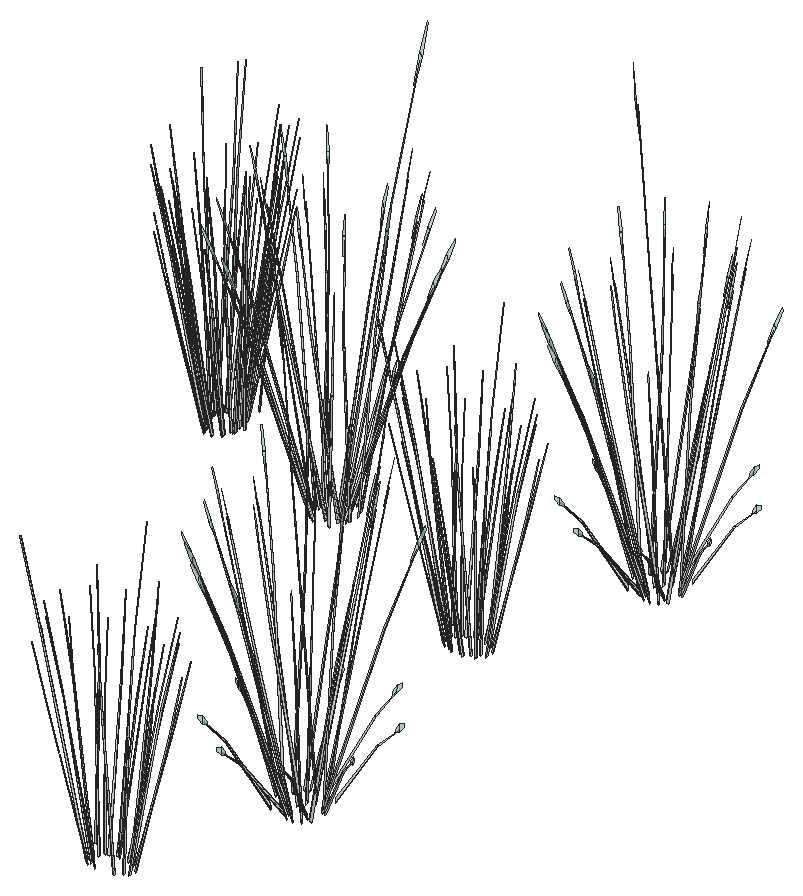
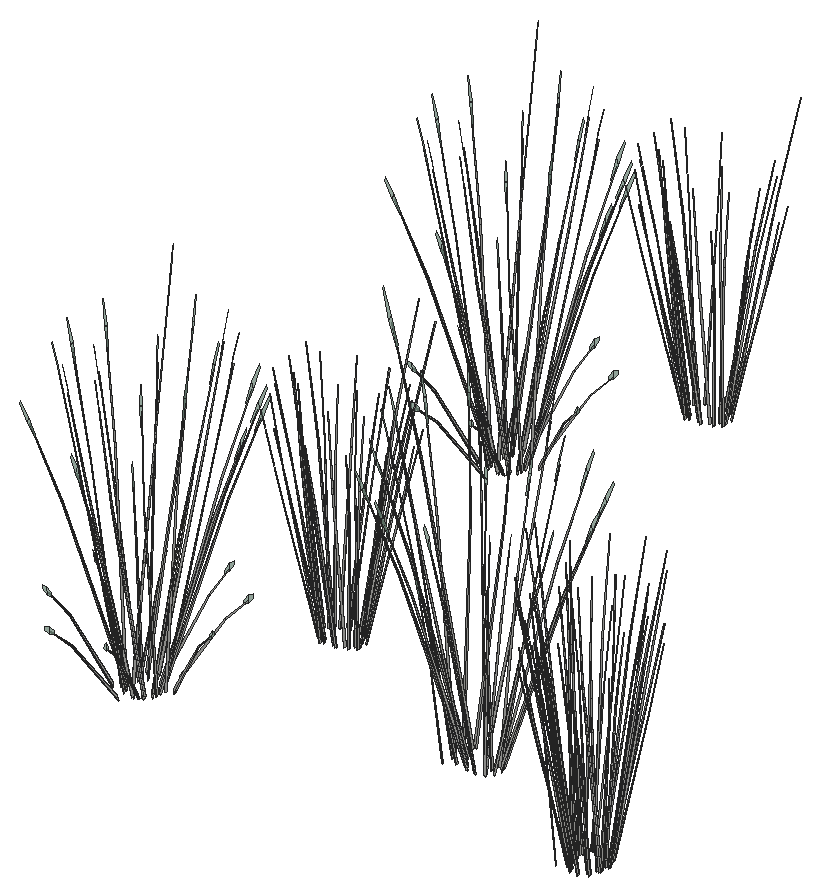
# SketchUp Ruby script. Lengths in inches.
U = 1.inch
M = Sketchup.active_model
def pt(a) = Geom::Point3d.new(a.map { |v| v * U })
def face(e, loops, mat)
  f = e.add_face(loops[0].map { |a| pt(a) })
  loops[1..].each { |l| e.add_face(l.map { |a| pt(a) }).erase! }
  f.material = f.back_material = mat if mat
  f
end
# faces: each face lists its corners as indices into pts; further lists are holes
def faces(e, pts, list, mat = nil) = list.each { |f| face(e, (f[0].is_a?(Array) ? f : [f]).map { |l| l.map { |i| pts[i] } }, mat) }
# xy, xz, yz: faces in a plane at the given z, y or x. An outline is a flat list of corners, or four numbers for a rectangle; further outlines are holes
def ring(l) = l.size == 4 ? [[l[0], l[1]], [l[2], l[1]], [l[2], l[3]], [l[0], l[3]]] : l.each_slice(2).to_a
def flat(e, list, mat, &to3) = list.each { |f| face(e, (f[0].is_a?(Array) ? f : [f]).map { |l| ring(l).map { |u, v| to3.(u, v) } }, mat) }
def xy(e, z, list, mat = nil) = flat(e, list, mat) { |x, y| [x, y, z] }
def xz(e, y, list, mat = nil) = flat(e, list, mat) { |x, z| [x, y, z] }
def yz(e, x, list, mat = nil) = flat(e, list, mat) { |y, z| [x, y, z] }
def lines(e, pts, list) = list.each { |a, b| e.add_line(pt(pts[a]), pt(pts[b])) }
# prism: a flat outline (further loops are holes) pulled along v
def prism(e, loops, v, mat = nil)
  f = face(e, loops, mat); d = Geom::Vector3d.new(v.map { |x| x * U })
  f.pushpull(f.normal.samedirection?(d) ? d.length : -d.length)
end
def box(e, o, s, mat = nil) = prism(e, [[o, [o[0] + s[0], o[1], o[2]], [o[0] + s[0], o[1] + s[1], o[2]], [o[0], o[1] + s[1], o[2]]]], [0, 0, s[2]], mat)
def at(x, y, z, deg = 0) = Geom::Transformation.translation(pt([x, y, z])) * Geom::Transformation.rotation(ORIGIN, Z_AXIS, deg.degrees)
def axes(o, x, y, z) = Geom::Transformation.new([*x, 0, *y, 0, *z, 0, *pt(o).to_a, 1])
def part(name) = M.definitions.add(name)
# library, detail: a bought-in or finely detailed component or shape, given as its bounding box
def library(name, o, s) = part(name).tap { |d| box(d.entities, o, s) }
def detail(e, o, s) = box(e.add_group.entities, o, s)
def put(e, d, t, mat = nil) = e.add_instance(d, t).tap { |i| i.material = mat if mat }
def group(e, t, mat = nil) = e.add_group.tap { |g| g.transformation = t; g.material = mat if mat }.entities
root = M.entities
M.materials.add("LightPink_Translucent").color = [175, 214, 192]
M.materials["LightPink_Translucent"].alpha = 0.75
c1 = part("blade")
p = [[2.15,0.21,22],[0,0.17,0],[0.09,0.45,0],[2.18,0.31,22],[2.29,0.31,22],[0.38,0.45,0],
  [2.48,0.24,33],[2.49,0.24,33],[2.48,0.22,33]]
faces(c1.entities,p,[[0,1,2,3],[4,5,2,3],[6,3,4,7],[8,0,3,6]])
c2 = part("blade with seeds\#1")
put(c2.entities,c1,at(0,0,0))
c3 = part("seeds")
p = [[0.3,-0.1,1.38],[-0.01,-0.03,1.59],[-0.01,-0.03,0.03],[0.14,-0.07,-0.07],[0.29,-0.03,3],[0.15,0.01,3.11]]
faces(c3.entities,p,[[0,1,2,3],[1,0,4,5]],"LightPink_Translucent")
c4 = part("blade with seeds")
put(c4.entities,c1,at(0,0,0))
put(c4.entities,c3,axes([2.4,0.25,30.99],[1.5799,-0.05474,1.17369],[-0.12525,1.92788,0.29478],[-0.07173,-0.02425,1.56792]))
put(root,c2,axes([487.46,499.57,140.86],[-0.33637,0.20062,0.29052],[-0.31842,-0.22908,-0.37506],[0.04845,-0.11639,0.71765]))
put(root,c2,axes([485.47,499.29,140.86],[0.07678,0.30692,0.29052],[-0.43892,0.08104,-0.37506],[-0.11789,-0.08795,0.71765]))
put(root,c2,axes([484.15,499.49,140.9],[0.41055,-0.28121,0.44104],[0.35407,0.29863,0.36366],[-0.19262,-0.05187,0.91263]))
put(root,c2,axes([484.34,499.49,140.6],[0.02503,-0.28975,0.05275],[0.378,0.00794,0.41527],[-0.1448,-0.03032,0.63322]))
put(root,c2,axes([488.05,500.19,140.86],[-0.43273,0.05446,0.29052],[-0.11427,-0.31131,-0.37506],[0.12401,-0.08362,0.71765]))
put(root,c2,axes([488.44,500.14,140.6],[0.34128,0.16025,0.05275],[-0.1987,0.22821,0.41527],[0.10942,-0.07378,0.63322]))
put(root,c2,axes([484.6,499.71,140.86],[0.28286,0.23857,0.29052],[-0.32298,0.22584,-0.37506],[-0.1641,-0.03436,0.71765]))
put(root,c2,axes([488.12,500.9375,140.86],[-0.41315,-0.1063,0.29052],[0.1205,-0.31012,-0.37506],[0.16634,-0.02844,0.71765]))
put(root,c2,axes([483.76,500.28,140.6],[-0.18259,-0.25981,0.05275],[0.33295,-0.12717,0.41527],[-0.14677,0.02509,0.63322]))
put(root,c2,axes([488.49,501.03,140.6],[0.18259,0.25981,0.05275],[-0.33295,0.12717,0.41527],[0.14677,-0.02509,0.63322]))
put(root,c2,axes([484.13,500.375,140.86],[0.41315,0.1063,0.29052],[-0.1205,0.31012,-0.37506],[-0.16634,0.02844,0.71765]))
put(root,c2,axes([487.65,501.61,140.86],[-0.28286,-0.23857,0.29052],[0.32298,-0.22584,-0.37506],[0.1641,0.03436,0.71765]))
put(root,c2,axes([483.81,501.17,140.6],[-0.34128,-0.16025,0.05275],[0.1987,-0.22821,0.41527],[-0.10942,0.07378,0.63322]))
put(root,c2,axes([484.2,501.12,140.86],[0.43273,-0.05446,0.29052],[0.11427,0.31131,-0.37506],[-0.12401,0.08362,0.71765]))
put(root,c2,axes([487.91,501.82,140.6],[-0.02503,0.28975,0.05275],[-0.378,-0.00794,0.41527],[0.1448,0.03032,0.63322]))
put(root,c2,axes([483.22,502,141.35],[0.43869,0.10171,-0.05322],[-0.13494,0.31305,-0.24131],[-0.07175,0.04753,0.79594]))
put(root,c2,axes([486.78,502.02,140.86],[-0.07678,-0.30692,0.29052],[0.43892,-0.08104,-0.37506],[0.11789,0.08795,0.71765]))
put(root,c2,axes([484.79,501.74,140.86],[0.33637,-0.20062,0.29052],[0.31842,0.22908,-0.37506],[-0.04845,0.11639,0.71765]))
put(root,c2,axes([484.48,501.92,140.6],[-0.40853,-0.01775,0.05275],[0.0112,-0.2681,0.41527],[-0.04275,0.1027,0.63322]))
put(root,c2,axes([485.73,502.07,140.86],[0.14987,-0.29303,0.29052],[0.43725,0.08547,-0.37506],[0.04009,0.11798,0.71765]))
put(root,c2,axes([486.85,502.3,140.6],[-0.22594,0.24206,0.05275],[-0.32175,-0.14093,0.41527],[0.10402,0.07761,0.63322]))
put(root,c2,axes([486.32,503.11,141.35],[0.34354,-0.2186,-0.05322],[0.31478,0.23941,-0.24131],[0.02216,0.06784,0.79594]))
put(root,c2,axes([485.59,502.33,140.6],[-0.36632,0.1295,0.05275],[-0.1793,-0.23615,0.41527],[0.03538,0.1041,0.63322]))
put(root,c2,axes([485.72,502.31,140.87],[-0.48986,-0.09962,0.43711],[0.16751,-0.3275,0.36041],[0.02944,0.12879,0.90448]))
put(root,c4,axes([493.6875,516.23,140.7],[0.01009,0.19824,1.55952],[-0.43714,-0.13151,0.1261],[0.02704,-0.28251,0.66668]))
put(root,c4,axes([492.92,516.3125,140.7],[0.0942,0.16583,1.55952],[-0.43527,0.13961,0.1261],[-0.09838,-0.26034,0.66668]))
put(root,c4,axes([493.07,515.81,141.46],[-0.05782,-0.07805,1.59199],[-0.42244,0.00664,-0.25177],[-0.05494,-0.1789,0.12768]))
put(root,c4,axes([494.39,516.61,140.7],[-0.07673,0.17753,1.55952],[-0.32188,-0.36739,0.1261],[0.14521,-0.22898,0.66668]))
put(root,c4,axes([495.1,516.57,141.46],[0.00314,-0.10283,1.59199],[-0.31434,-0.32739,-0.25177],[0.06423,-0.17468,0.12768]))
put(root,c4,axes([493.47,516.31,141.75],[-0.40325,0.24047,-0.11066],[-0.19816,-0.4268,-0.6142],[-0.0532,-0.17986,0.93327]))
put(root,c4,axes([494.3125,516.85,141.75],[-0.45289,-0.02559,-0.11066],[0.01238,-0.48454,-0.6142],[0.03146,-0.18661,0.93327]))
put(root,c4,axes([492.625,516.92,140.7],[0.13683,0.11937,1.55952],[-0.36934,0.30141,0.1261],[-0.1682,-0.20674,0.66668]))
put(root,c4,axes([492.29,516.83,140.7],[0.15307,0.08899,1.55952],[-0.31677,0.37333,0.1261],[-0.19743,-0.16841,0.66668]))
put(root,c4,axes([491.49,515.82,141.46],[-0.08813,-0.01188,1.59199],[-0.30658,0.33715,-0.25177],[-0.14498,-0.08826,0.12768]))
put(root,c4,axes([492.51,516.33,141.75],[-0.24556,0.44211,-0.11066],[-0.35561,-0.2547,-0.6142],[-0.12361,-0.12491,0.93327]))
put(root,c4,axes([494.83,517.34,140.7],[-0.14298,0.10925,1.55952],[-0.12037,-0.50484,0.1261],[0.22447,-0.1141,0.66668]))
put(root,c4,axes([495.78,518.17,141.46],[0.06244,-0.0731,1.59199],[-0.03959,-0.48785,-0.25177],[0.14934,-0.07786,0.12768]))
put(root,c4,axes([494.82,518.91,141.75],[-0.20734,-0.4677,-0.11066],[0.36799,-0.22984,-0.6142],[0.15507,-0.06171,0.93327]))
put(root,c4,axes([491.96,517.64,140.7],[0.17092,-0.0117,1.55952],[-0.11339,0.50701,0.1261],[-0.24358,-0.03136,0.66668]))
put(root,c4,axes([490.4,517.76,141.46],[-0.07171,0.06058,1.59199],[-0.02817,0.48891,-0.25177],[-0.15815,0.04916,0.12768]))
put(root,c4,axes([491.23,517.87,141.75],[0.20734,0.4677,-0.11066],[-0.36799,0.22984,-0.6142],[-0.15507,0.06171,0.93327]))
put(root,c4,axes([494.35,519.88,141.75],[0.02206,-0.52527,-0.11066],[0.41777,0.01436,-0.6142],[0.1609,0.03649,0.93327]))
put(root,c4,axes([492.04,518.54,140.7],[0.14298,-0.10925,1.55952],[0.12037,0.50484,0.1261],[-0.22447,0.1141,0.66668]))
put(root,c4,axes([493.49,519.3,141.24],[0.23139,-0.41299,1.25837],[0.36026,0.43608,0.54295],[-0.21711,0.13325,1.21634]))
put(root,c4,axes([495.02,520.36,141.46],[0.08863,-0.00461,1.59199],[0.25616,-0.38966,-0.25177],[0.15528,0.06024,0.12768]))
put(root,c4,axes([494.58,519.04,140.7],[-0.15307,-0.08899,1.55952],[0.31677,-0.37333,0.1261],[0.19743,0.16841,0.66668]))
put(root,c4,axes([491.24,518.98,141.75],[0.38119,0.2848,-0.11066],[-0.21961,0.41244,-0.6142],[-0.10769,0.14337,0.93327]))
put(root,c4,axes([493.53,520.46,141.75],[0.24556,-0.44211,-0.11066],[0.35561,0.2547,-0.6142],[0.12361,0.12491,0.93327]))
put(root,c4,axes([492.48,519.27,140.7],[0.07673,-0.17753,1.55952],[0.32188,0.36739,0.1261],[-0.14521,0.22898,0.66668]))
put(root,c4,axes([491.73,519.93,141.75],[0.45289,0.02559,-0.11066],[-0.01238,0.48454,-0.6142],[-0.03146,0.18661,0.93327]))
put(root,c4,axes([492.57,520.47,141.75],[0.40325,-0.24047,-0.11066],[0.19816,0.4268,-0.6142],[0.0532,0.17986,0.93327]))
put(root,c4,axes([492.01,520.36,141.46],[0.00753,0.10253,1.59199],[0.34598,0.28122,-0.25177],[-0.04567,0.18237,0.12768]))
put(root,c4,axes([493.18,519.64,140.7],[-0.01009,-0.19824,1.55952],[0.43714,0.13151,0.1261],[-0.02704,0.28251,0.66668]))
put(root,c4,axes([493.2,521.78,141.46],[0.06783,0.06632,1.59199],[0.4161,-0.08489,-0.25177],[0.07889,0.16641,0.12768]))
put(root,c2,axes([485.28,547.98,140.9],[0.55379,-0.09794,0.44104],[0.09611,0.38419,0.36366],[-0.13024,-0.11323,0.91263]))
put(root,c2,axes([486.66,548.03,140.6],[0.36632,-0.1295,0.05275],[0.1793,0.23615,0.41527],[-0.03538,-0.1041,0.63322]))
put(root,c2,axes([485.4,548.0625,140.6],[0.22594,-0.24206,0.05275],[0.32175,0.14093,0.41527],[-0.10402,-0.07761,0.63322]))
put(root,c2,axes([486.52,548.29,140.86],[-0.14987,0.29303,0.29052],[-0.43725,-0.08547,-0.37506],[-0.04009,-0.11798,0.71765]))
put(root,c2,axes([487.77,548.4375,140.6],[0.40853,0.01775,0.05275],[-0.0112,0.2681,0.41527],[0.04275,-0.1027,0.63322]))
put(root,c2,axes([487.46,548.62,140.86],[-0.33637,0.20062,0.29052],[-0.31842,-0.22908,-0.37506],[0.04845,-0.11639,0.71765]))
put(root,c2,axes([485.47,548.34,140.86],[0.07678,0.30692,0.29052],[-0.43892,0.08104,-0.37506],[-0.11789,-0.08795,0.71765]))
put(root,c2,axes([484.15,548.54,140.9],[0.41055,-0.28121,0.44104],[0.35407,0.29863,0.36366],[-0.19262,-0.05187,0.91263]))
put(root,c2,axes([484.34,548.54,140.6],[0.02503,-0.28975,0.05275],[0.378,0.00794,0.41527],[-0.1448,-0.03032,0.63322]))
put(root,c2,axes([488.05,549.24,140.86],[-0.43273,0.05446,0.29052],[-0.11427,-0.31131,-0.37506],[0.12401,-0.08362,0.71765]))
put(root,c2,axes([488.44,549.19,140.6],[0.34128,0.16025,0.05275],[-0.1987,0.22821,0.41527],[0.10942,-0.07378,0.63322]))
put(root,c2,axes([484.6,548.75,140.86],[0.28286,0.23857,0.29052],[-0.32298,0.22584,-0.37506],[-0.1641,-0.03436,0.71765]))
put(root,c2,axes([488.12,549.99,140.86],[-0.41315,-0.1063,0.29052],[0.1205,-0.31012,-0.37506],[0.16634,-0.02844,0.71765]))
put(root,c2,axes([483.76,549.33,140.6],[-0.18259,-0.25981,0.05275],[0.33295,-0.12717,0.41527],[-0.14677,0.02509,0.63322]))
put(root,c2,axes([488.49,550.08,140.6],[0.18259,0.25981,0.05275],[-0.33295,0.12717,0.41527],[0.14677,-0.02509,0.63322]))
put(root,c2,axes([484.13,549.42,140.86],[0.41315,0.1063,0.29052],[-0.1205,0.31012,-0.37506],[-0.16634,0.02844,0.71765]))
put(root,c2,axes([487.65,550.65,140.86],[-0.28286,-0.23857,0.29052],[0.32298,-0.22584,-0.37506],[0.1641,0.03436,0.71765]))
put(root,c2,axes([483.81,550.22,140.6],[-0.34128,-0.16025,0.05275],[0.1987,-0.22821,0.41527],[-0.10942,0.07378,0.63322]))
put(root,c2,axes([484.2,550.17,140.86],[0.43273,-0.05446,0.29052],[0.11427,0.31131,-0.37506],[-0.12401,0.08362,0.71765]))
put(root,c2,axes([487.91,550.87,140.6],[-0.02503,0.28975,0.05275],[-0.378,-0.00794,0.41527],[0.1448,0.03032,0.63322]))
put(root,c2,axes([483.22,551.05,141.35],[0.43869,0.10171,-0.05322],[-0.13494,0.31305,-0.24131],[-0.07175,0.04753,0.79594]))
put(root,c2,axes([486.78,551.07,140.86],[-0.07678,-0.30692,0.29052],[0.43892,-0.08104,-0.37506],[0.11789,0.08795,0.71765]))
put(root,c2,axes([484.79,550.79,140.86],[0.33637,-0.20062,0.29052],[0.31842,0.22908,-0.37506],[-0.04845,0.11639,0.71765]))
put(root,c2,axes([484.48,550.97,140.6],[-0.40853,-0.01775,0.05275],[0.0112,-0.2681,0.41527],[-0.04275,0.1027,0.63322]))
put(root,c2,axes([485.73,551.12,140.86],[0.14987,-0.29303,0.29052],[0.43725,0.08547,-0.37506],[0.04009,0.11798,0.71765]))
put(root,c2,axes([486.85,551.35,140.6],[-0.22594,0.24206,0.05275],[-0.32175,-0.14093,0.41527],[0.10402,0.07761,0.63322]))
put(root,c2,axes([486.32,552.16,141.35],[0.34354,-0.2186,-0.05322],[0.31478,0.23941,-0.24131],[0.02216,0.06784,0.79594]))
put(root,c2,axes([485.59,551.38,140.6],[-0.36632,0.1295,0.05275],[-0.1793,-0.23615,0.41527],[0.03538,0.1041,0.63322]))
put(root,c2,axes([485.72,551.36,140.87],[-0.48986,-0.09962,0.43711],[0.16751,-0.3275,0.36041],[0.02944,0.12879,0.90448]))
put(root,c4,axes([462.24,558.24,140.79],[0.10925,0.14298,1.55952],[-0.50484,0.12037,0.1261],[-0.1141,-0.22447,0.66668]))
put(root,c4,axes([463.95,558.49,140.79],[-0.08899,0.15307,1.55952],[-0.37333,-0.31677,0.1261],[0.16841,-0.19743,0.66668]))
put(root,c4,axes([463.82,558.25,141.85],[-0.4677,0.20734,-0.11066],[-0.22984,-0.36799,-0.6142],[-0.06171,-0.15507,0.93327]))
put(root,c4,axes([464.79,558.72,141.85],[-0.52527,-0.02206,-0.11066],[0.01436,-0.41777,-0.6142],[0.03649,-0.1609,0.93327]))
put(root,c4,axes([461.51,558.68,140.79],[0.17753,0.07673,1.55952],[-0.36739,0.32188,0.1261],[-0.22898,-0.14521,0.66668]))
put(root,c4,axes([465.36,559.54,141.85],[-0.44211,-0.24556,-0.11066],[0.2547,-0.35561,-0.6142],[0.12491,-0.12361,0.93327]))
put(root,c4,axes([461.75,558.76,141.85],[-0.02559,0.45289,-0.11066],[-0.48454,-0.01238,-0.6142],[-0.18661,-0.03146,0.93327]))
put(root,c4,axes([465.38,560.5,141.85],[-0.24047,-0.40325,-0.11066],[0.4268,-0.19816,-0.6142],[0.17986,-0.0532,0.93327]))
put(root,c4,axes([461.14,559.38,140.79],[0.19824,-0.01009,1.55952],[-0.13151,0.43714,0.1261],[-0.28251,-0.02704,0.66668]))
put(root,c4,axes([464.55,559.89,140.79],[-0.19824,0.01009,1.55952],[0.13151,-0.43714,0.1261],[0.28251,0.02704,0.66668]))
put(root,c4,axes([493.6875,565.28,140.7],[0.01009,0.19824,1.55952],[-0.43714,-0.13151,0.1261],[0.02704,-0.28251,0.66668]))
put(root,c4,axes([492.92,565.36,140.7],[0.0942,0.16583,1.55952],[-0.43527,0.13961,0.1261],[-0.09838,-0.26034,0.66668]))
put(root,c4,axes([461.21,559.6,141.85],[0.24047,0.40325,-0.11066],[-0.4268,0.19816,-0.6142],[-0.17986,0.0532,0.93327]))
put(root,c4,axes([465.96,561.35,140.84],[-0.09148,-0.37435,-0.03177],[0.43236,-0.08606,-0.14407],[0.09029,0.02373,0.47519]))
put(root,c4,axes([464.84,561.34,141.85],[0.02559,-0.45289,-0.11066],[0.48454,0.01238,-0.6142],[0.18661,0.03146,0.93327]))
put(root,c4,axes([493.07,564.86,141.46],[-0.05782,-0.07805,1.59199],[-0.42244,0.00664,-0.25177],[-0.05494,-0.1789,0.12768]))
put(root,c4,axes([494.39,565.65,140.7],[-0.07673,0.17753,1.55952],[-0.32188,-0.36739,0.1261],[0.14521,-0.22898,0.66668]))
put(root,c4,axes([461.22,560.15,140.79],[0.16583,-0.0942,1.55952],[0.13961,0.43527,0.1261],[-0.26034,0.09838,0.66668]))
put(root,c2,axes([445.85,564.61,140.7],[0.34743,0.14045,0.39379],[-0.1188,0.46175,0.3247],[-0.02088,-0.18159,0.81485]))
put(root,c2,axes([445.94,564.58,140.69],[0.25981,-0.18259,0.05275],[0.12717,0.33295,0.41527],[-0.02509,-0.14677,0.63322]))
put(root,c4,axes([495.1,565.62,141.46],[0.00314,-0.10283,1.59199],[-0.31434,-0.32739,-0.25177],[0.06423,-0.17468,0.12768]))
put(root,c4,axes([493.47,565.36,141.75],[-0.40325,0.24047,-0.11066],[-0.19816,-0.4268,-0.6142],[-0.0532,-0.17986,0.93327]))
put(root,c2,axes([444.98,564.72,140.7],[0.35069,-0.12329,0.39379],[0.06086,0.48364,0.3247],[-0.08248,-0.14254,0.81485]))
put(root,c4,axes([494.3125,565.9,141.75],[-0.45289,-0.02559,-0.11066],[0.01238,-0.48454,-0.6142],[0.03146,-0.18661,0.93327]))
put(root,c2,axes([445.05,564.63,140.69],[0.16025,-0.34128,0.05275],[0.22821,0.1987,0.41527],[-0.07378,-0.10942,0.63322]))
put(root,c4,axes([492.625,565.97,140.7],[0.13683,0.11937,1.55952],[-0.36934,0.30141,0.1261],[-0.1682,-0.20674,0.66668]))
put(root,c2,axes([445.84,564.95,140.96],[-0.1063,0.41315,0.29052],[-0.31012,-0.1205,-0.37506],[-0.02844,-0.16634,0.71765]))
put(root,c2,axes([446.64,565.13,140.7],[0.25108,0.36656,0.39379],[-0.26664,0.31614,0.3247],[0.04631,-0.17198,0.81485]))
put(root,c2,axes([446.73,565.16,140.69],[0.28975,0.02503,0.05275],[-0.00794,0.378,0.41527],[0.03032,-0.1448,0.63322]))
put(root,c2,axes([446.51,565.42,140.96],[-0.23857,0.28286,0.29052],[-0.22584,-0.32298,-0.37506],[0.03436,-0.1641,0.71765]))
put(root,c4,axes([492.29,565.88,140.7],[0.15307,0.08899,1.55952],[-0.31677,0.37333,0.1261],[-0.19743,-0.16841,0.66668]))
put(root,c4,axes([464.18,560.59,140.79],[-0.17753,-0.07673,1.55952],[0.36739,-0.32188,0.1261],[0.22898,0.14521,0.66668]))
put(root,c4,axes([464.21,559.58,141.34],[-0.41299,-0.23139,1.25837],[0.43608,-0.36026,0.54295],[0.13325,0.21711,1.21634]))
put(root,c4,axes([461.23,560.56,141.85],[0.44211,0.24556,-0.11066],[-0.2547,0.35561,-0.6142],[-0.12491,0.12361,0.93327]))
put(root,c4,axes([463.89,561.83,141.85],[0.2848,-0.38119,-0.11066],[0.41244,0.21961,-0.6142],[0.14337,0.10769,0.93327]))
put(root,c4,axes([491.49,564.87,141.46],[-0.08813,-0.01188,1.59199],[-0.30658,0.33715,-0.25177],[-0.14498,-0.08826,0.12768]))
put(root,c4,axes([461.83,560.45,140.79],[0.11937,-0.13683,1.55952],[0.30141,0.36934,0.1261],[-0.20674,0.1682,0.66668]))
put(root,c2,axes([445.1,565.02,140.96],[0.05446,0.43273,0.29052],[-0.31131,0.11427,-0.37506],[-0.08362,-0.12401,0.71765]))
put(root,c4,axes([492.51,565.375,141.75],[-0.24556,0.44211,-0.11066],[-0.35561,-0.2547,-0.6142],[-0.12361,-0.12491,0.93327]))
put(root,c2,axes([444.27,565.43,140.7],[0.25999,-0.354,0.39379],[0.22422,0.37594,0.3247],[-0.12198,-0.0653,0.81485]))
put(root,c2,axes([444.3,565.3,140.69],[0.01775,-0.40853,0.05275],[0.2681,0.0112,0.41527],[-0.1027,-0.04275,0.63322]))
put(root,c4,axes([461.74,560.78,140.79],[0.08899,-0.15307,1.55952],[0.37333,0.31677,0.1261],[-0.16841,0.19743,0.66668]))
put(root,c2,axes([446.93,566.29,140.96],[-0.30692,0.07678,0.29052],[-0.08104,-0.43892,-0.37506],[0.08795,-0.11789,0.71765]))
put(root,c4,axes([494.83,566.39,140.7],[-0.14298,0.10925,1.55952],[-0.12037,-0.50484,0.1261],[0.22447,-0.1141,0.66668]))
put(root,c4,axes([462.78,561.84,141.85],[0.4677,-0.20734,-0.11066],[0.22984,0.36799,-0.6142],[0.06171,0.15507,0.93327]))
put(root,c2,axes([447.14,566.13,140.7],[0.08745,0.49445,0.39379],[-0.34303,0.08581,0.3247],[0.1011,-0.11629,0.81485]))
put(root,c4,axes([463.44,561.04,140.79],[-0.10925,-0.14298,1.55952],[0.50484,-0.12037,0.1261],[0.1141,0.22447,0.66668]))
put(root,c2,axes([447.21,566.22,140.69],[0.24206,0.22594,0.05275],[-0.14093,0.32175,0.41527],[0.07761,-0.10402,0.63322]))
put(root,c4,axes([462.55,561.11,140.79],[-0.0117,-0.17092,1.55952],[0.50701,0.11339,0.1261],[-0.03136,0.24358,0.66668]))
put(root,c2,axes([444.48,565.61,140.96],[0.20062,0.33637,0.29052],[-0.22908,0.31842,-0.37506],[-0.11639,-0.04845,0.71765]))
put(root,c4,axes([495.78,567.22,141.46],[0.06244,-0.0731,1.59199],[-0.03959,-0.48785,-0.25177],[0.14934,-0.07786,0.12768]))
put(root,c2,axes([448.02,566.75,141.44],[-0.2186,-0.34354,-0.05322],[0.23941,-0.31478,-0.24131],[0.06784,-0.02216,0.79594]))
put(root,c4,axes([494.82,567.96,141.75],[-0.20734,-0.4677,-0.11066],[0.36799,-0.22984,-0.6142],[0.15507,-0.06171,0.93327]))
put(root,c4,axes([491.96,566.69,140.7],[0.17092,-0.0117,1.55952],[-0.11339,0.50701,0.1261],[-0.24358,-0.03136,0.66668]))
put(root,c2,axes([446.98,567.34,140.96],[-0.29303,-0.14987,0.29052],[0.08547,-0.43725,-0.37506],[0.11798,-0.04009,0.71765]))
put(root,c2,axes([443.91,566.54,140.7],[0.09962,-0.48986,0.39379],[0.3275,0.16751,0.3247],[-0.12879,0.02944,0.81485]))
put(root,c2,axes([443.88,566.41,140.69],[-0.1295,-0.36632,0.05275],[0.23615,-0.1793,0.41527],[-0.1041,0.03538,0.63322]))
put(root,c2,axes([447.24,567.48,140.69],[0.1295,0.36632,0.05275],[-0.23615,0.1793,0.41527],[0.1041,-0.03538,0.63322]))
put(root,c2,axes([447.22,567.35,140.97],[-0.09962,0.48986,0.43711],[-0.3275,-0.16751,0.36041],[0.12879,-0.02944,0.90448]))
put(root,c2,axes([444.15,566.55,140.96],[0.29303,0.14987,0.29052],[-0.08547,0.43725,-0.37506],[-0.11798,0.04009,0.71765]))
put(root,c4,axes([490.4,566.81,141.46],[-0.07171,0.06058,1.59199],[-0.02817,0.48891,-0.25177],[-0.15815,0.04916,0.12768]))
put(root,c2,axes([446.7,568.5,141.24],[0.01888,-0.54637,-0.11073],[0.35746,0.01493,-0.6146],[0.13767,0.03795,0.93387]))
put(root,c2,axes([446.65,568.29,140.96],[-0.20062,-0.33637,0.29052],[0.22908,-0.31842,-0.37506],[0.11639,0.04845,0.71765]))
put(root,c4,axes([491.23,566.92,141.75],[0.20734,0.4677,-0.11066],[-0.36799,0.22984,-0.6142],[-0.15507,0.06171,0.93327]))
put(root,c4,axes([494.35,568.93,141.75],[0.02206,-0.52527,-0.11066],[0.41777,0.01436,-0.6142],[0.1609,0.03649,0.93327]))
put(root,c2,axes([443.92,567.67,140.69],[-0.24206,-0.22594,0.05275],[0.14093,-0.32175,0.41527],[-0.07761,0.10402,0.63322]))
put(root,c2,axes([443.84,567.8,140.99],[-0.09794,-0.55379,0.44104],[0.38419,-0.09611,0.36366],[-0.11323,0.13024,0.91263]))
put(root,c2,axes([444.2,567.6,140.96],[0.30692,-0.07678,0.29052],[0.08104,0.43892,-0.37506],[-0.08795,0.11789,0.71765]))
put(root,c4,axes([492.04,567.59,140.7],[0.14298,-0.10925,1.55952],[0.12037,0.50484,0.1261],[-0.22447,0.1141,0.66668]))
put(root,c2,axes([446.83,568.59,140.69],[-0.01775,0.40853,0.05275],[-0.2681,-0.0112,0.41527],[0.1027,0.04275,0.63322]))
put(root,c2,axes([446.85,568.46,140.7],[-0.25999,0.354,0.39379],[-0.22422,-0.37594,0.3247],[0.12198,0.0653,0.81485]))
put(root,c4,axes([493.49,568.35,141.24],[0.23139,-0.41299,1.25837],[0.36026,0.43608,0.54295],[-0.21711,0.13325,1.21634]))
put(root,c2,axes([446.03,568.87,140.96],[-0.05446,-0.43273,0.29052],[0.31131,-0.11427,-0.37506],[0.08362,0.12401,0.71765]))
put(root,c4,axes([495.02,569.41,141.46],[0.08863,-0.00461,1.59199],[0.25616,-0.38966,-0.25177],[0.15528,0.06024,0.12768]))
put(root,c2,axes([446.91,569.85,141.44],[0.10171,-0.43869,-0.05322],[0.31305,0.13494,-0.24131],[0.04753,0.07175,0.79594]))
put(root,c2,axes([443.89,567.57,141.27],[0.3653,0.33178,-0.11173],[-0.21045,0.48049,-0.62013],[-0.10321,0.16702,0.94228]))
put(root,c2,axes([444.61,568.47,140.96],[0.23857,-0.28286,0.29052],[0.22584,0.32298,-0.37506],[-0.03436,0.1641,0.71765]))
put(root,c4,axes([494.58,568.09,140.7],[-0.15307,-0.08899,1.55952],[0.31677,-0.37333,0.1261],[0.19743,0.16841,0.66668]))
put(root,c2,axes([444.4,568.73,140.69],[-0.28975,-0.02503,0.05275],[0.00794,-0.378,0.41527],[-0.03032,0.1448,0.63322]))
put(root,c4,axes([491.24,568.03,141.75],[0.38119,0.2848,-0.11066],[-0.21961,0.41244,-0.6142],[-0.10769,0.14337,0.93327]))
put(root,c4,axes([493.53,569.51,141.75],[0.24556,-0.44211,-0.11066],[0.35561,0.2547,-0.6142],[0.12361,0.12491,0.93327]))
put(root,c2,axes([445.28,568.9375,140.96],[0.1063,-0.41315,0.29052],[0.31012,0.1205,-0.37506],[0.02844,0.16634,0.71765]))
put(root,c2,axes([446.07,569.26,140.69],[-0.16025,0.34128,0.05275],[-0.22821,-0.1987,0.41527],[0.07378,0.10942,0.63322]))
put(root,c2,axes([444.4,568.92,140.99],[-0.28121,-0.41055,0.44104],[0.29863,-0.35407,0.36366],[-0.05187,0.19262,0.91263]))
put(root,c2,axes([446.14,569.17,140.7],[-0.35069,0.12329,0.39379],[-0.06086,-0.48364,0.3247],[0.08248,0.14254,0.81485]))
put(root,c2,axes([445.18,569.3125,140.69],[-0.25981,0.18259,0.05275],[-0.12717,-0.33295,0.41527],[0.02509,0.14677,0.63322]))
put(root,c2,axes([445.28,569.28,140.7],[-0.34743,-0.14045,0.39379],[0.1188,-0.46175,0.3247],[0.02088,0.18159,0.81485]))
put(root,c4,axes([492.48,568.32,140.7],[0.07673,-0.17753,1.55952],[0.32188,0.36739,0.1261],[-0.14521,0.22898,0.66668]))
put(root,c4,axes([491.73,568.98,141.75],[0.45289,0.02559,-0.11066],[-0.01238,0.48454,-0.6142],[-0.03146,0.18661,0.93327]))
put(root,c4,axes([492.57,569.52,141.75],[0.40325,-0.24047,-0.11066],[0.19816,0.4268,-0.6142],[0.0532,0.17986,0.93327]))
put(root,c4,axes([492.01,569.4,141.46],[0.00753,0.10253,1.59199],[0.34598,0.28122,-0.25177],[-0.04567,0.18237,0.12768]))
put(root,c4,axes([493.18,568.69,140.7],[-0.01009,-0.19824,1.55952],[0.43714,0.13151,0.1261],[-0.02704,0.28251,0.66668]))
put(root,c4,axes([493.2,570.83,141.46],[0.06783,0.06632,1.59199],[0.4161,-0.08489,-0.25177],[0.07889,0.16641,0.12768]))
